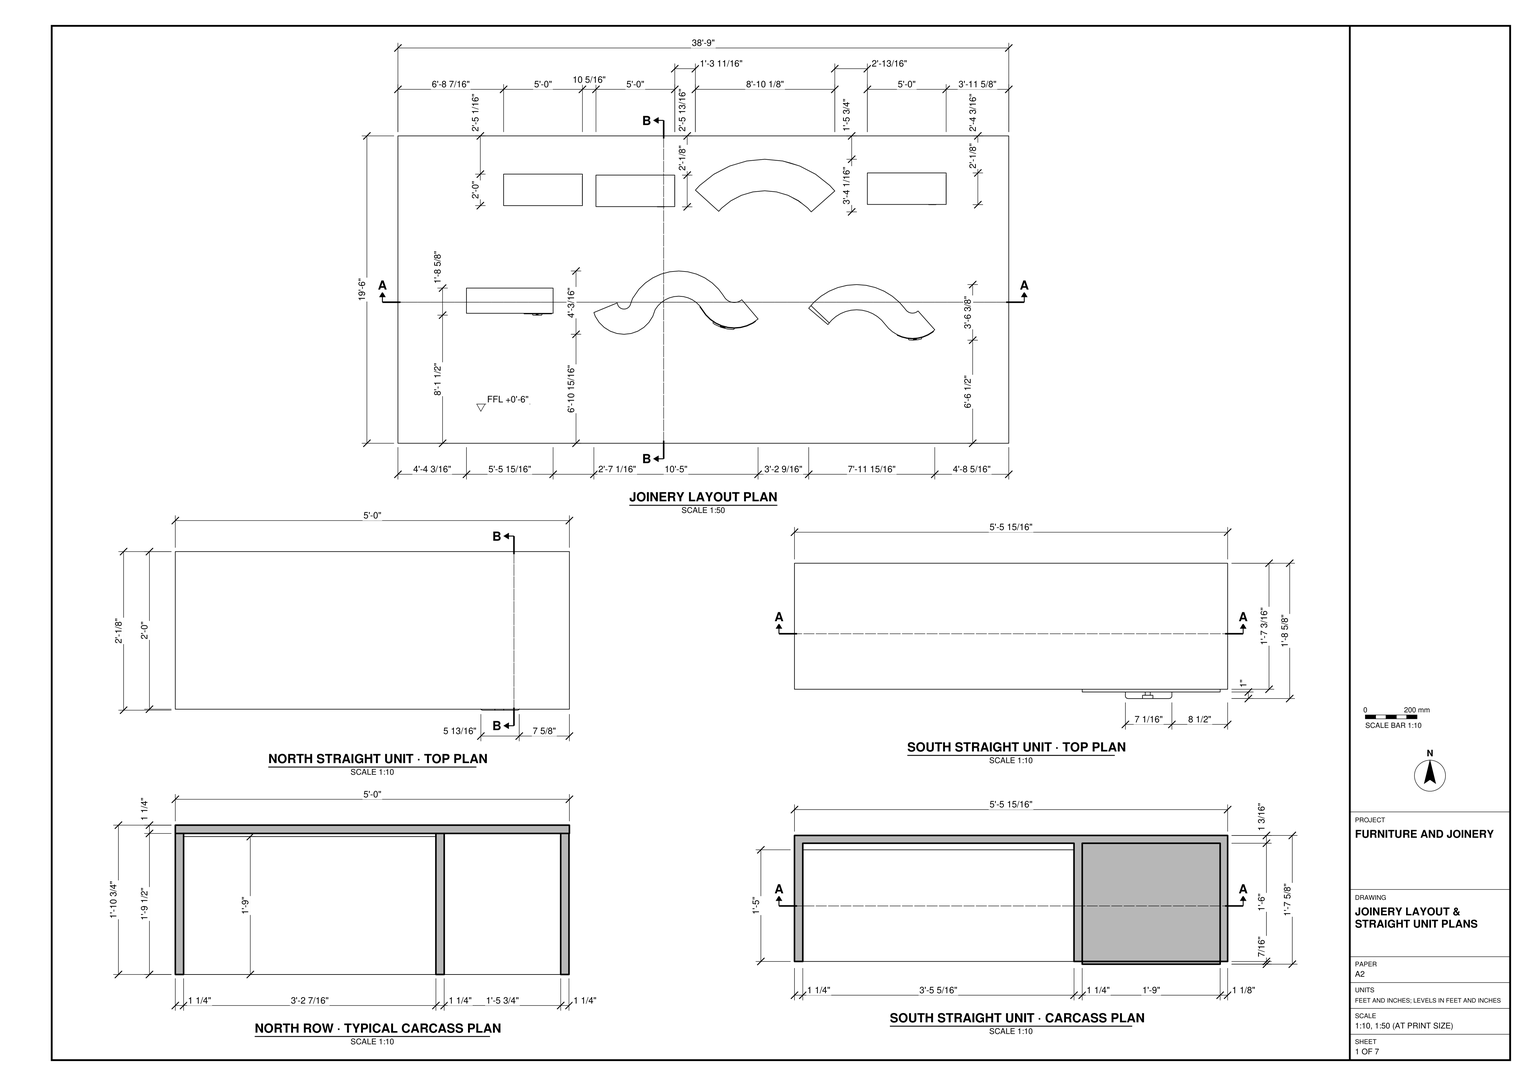
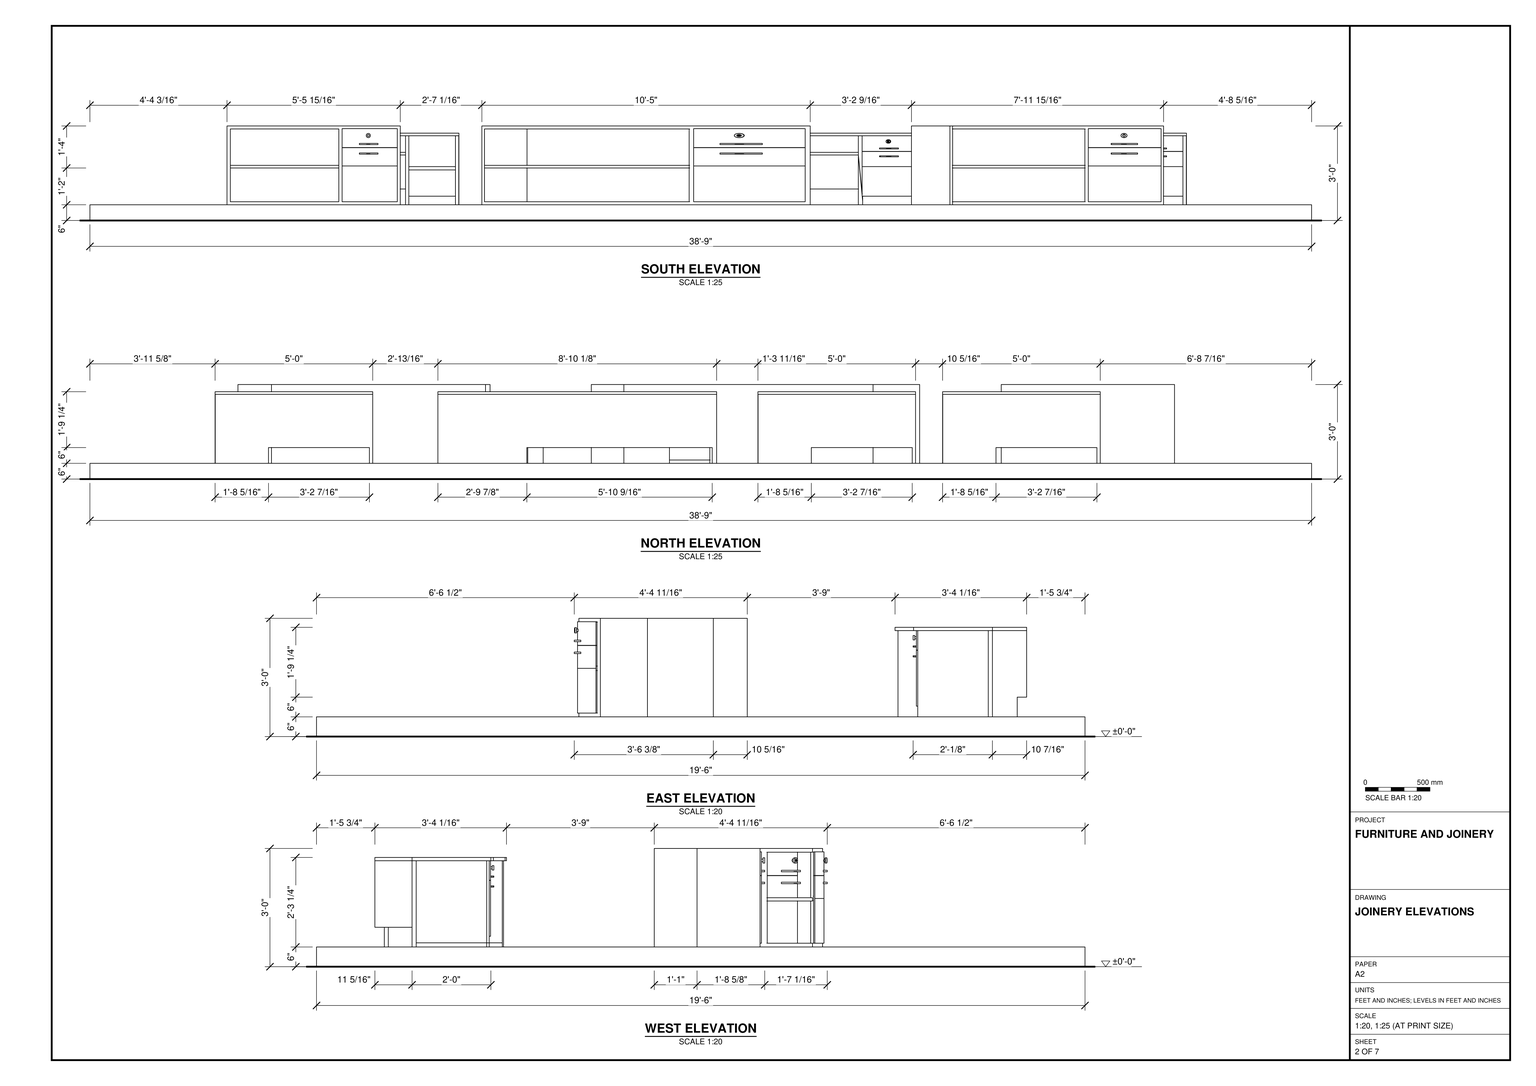
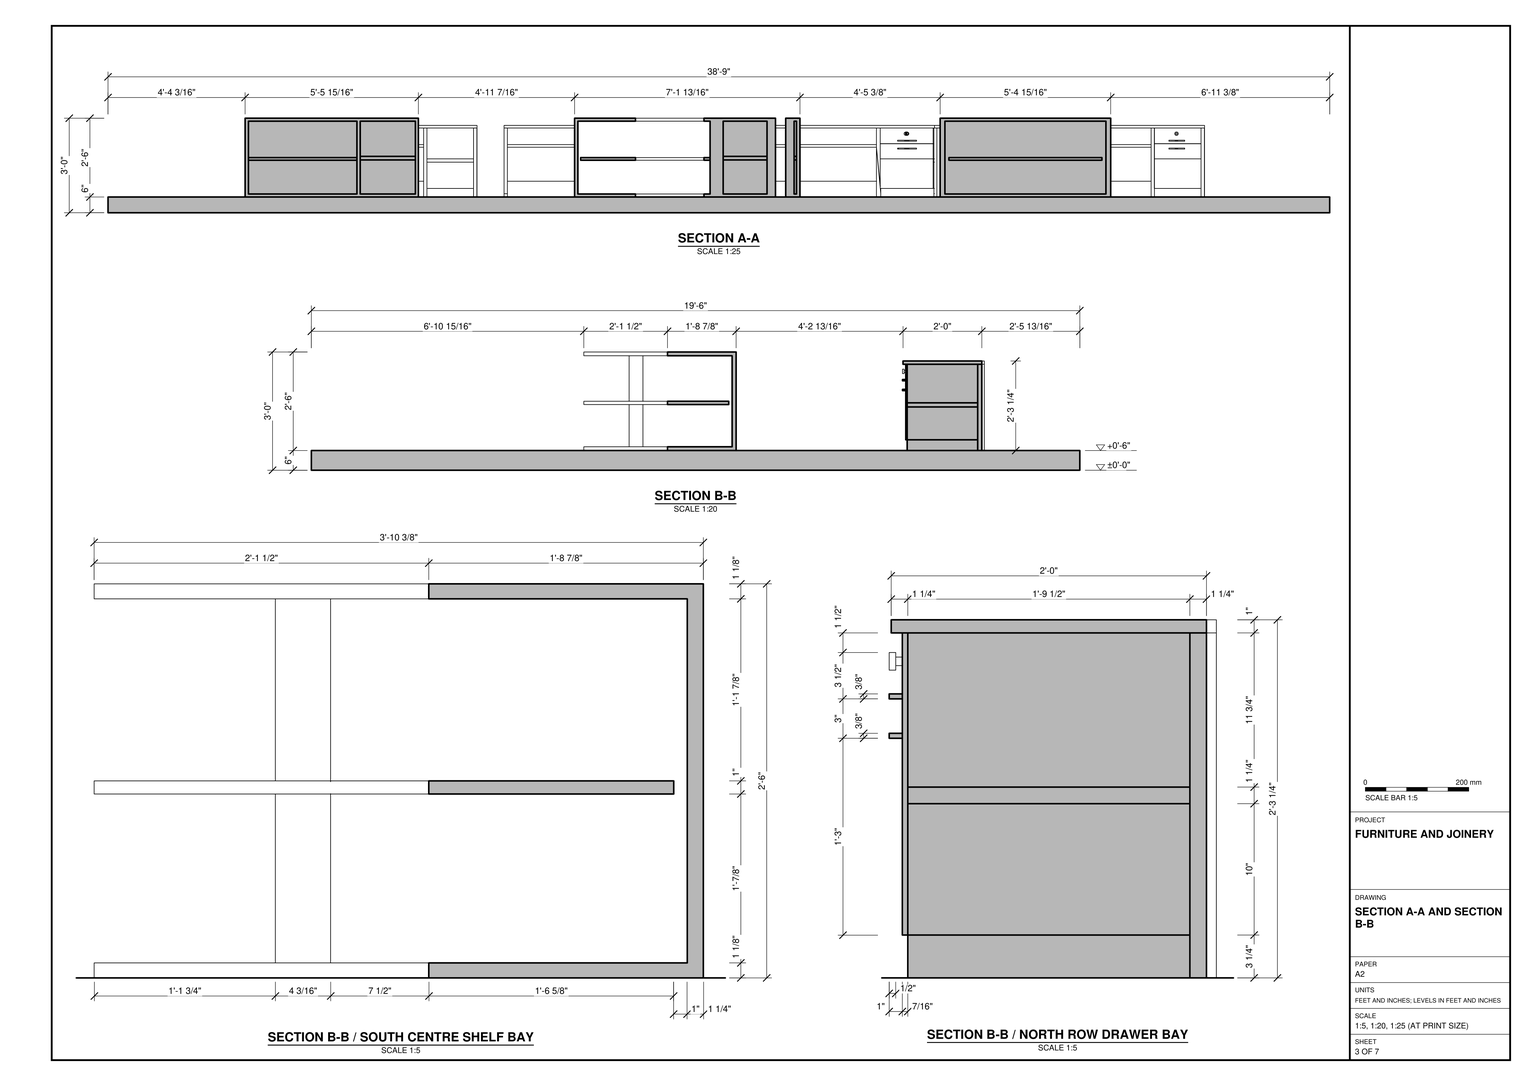
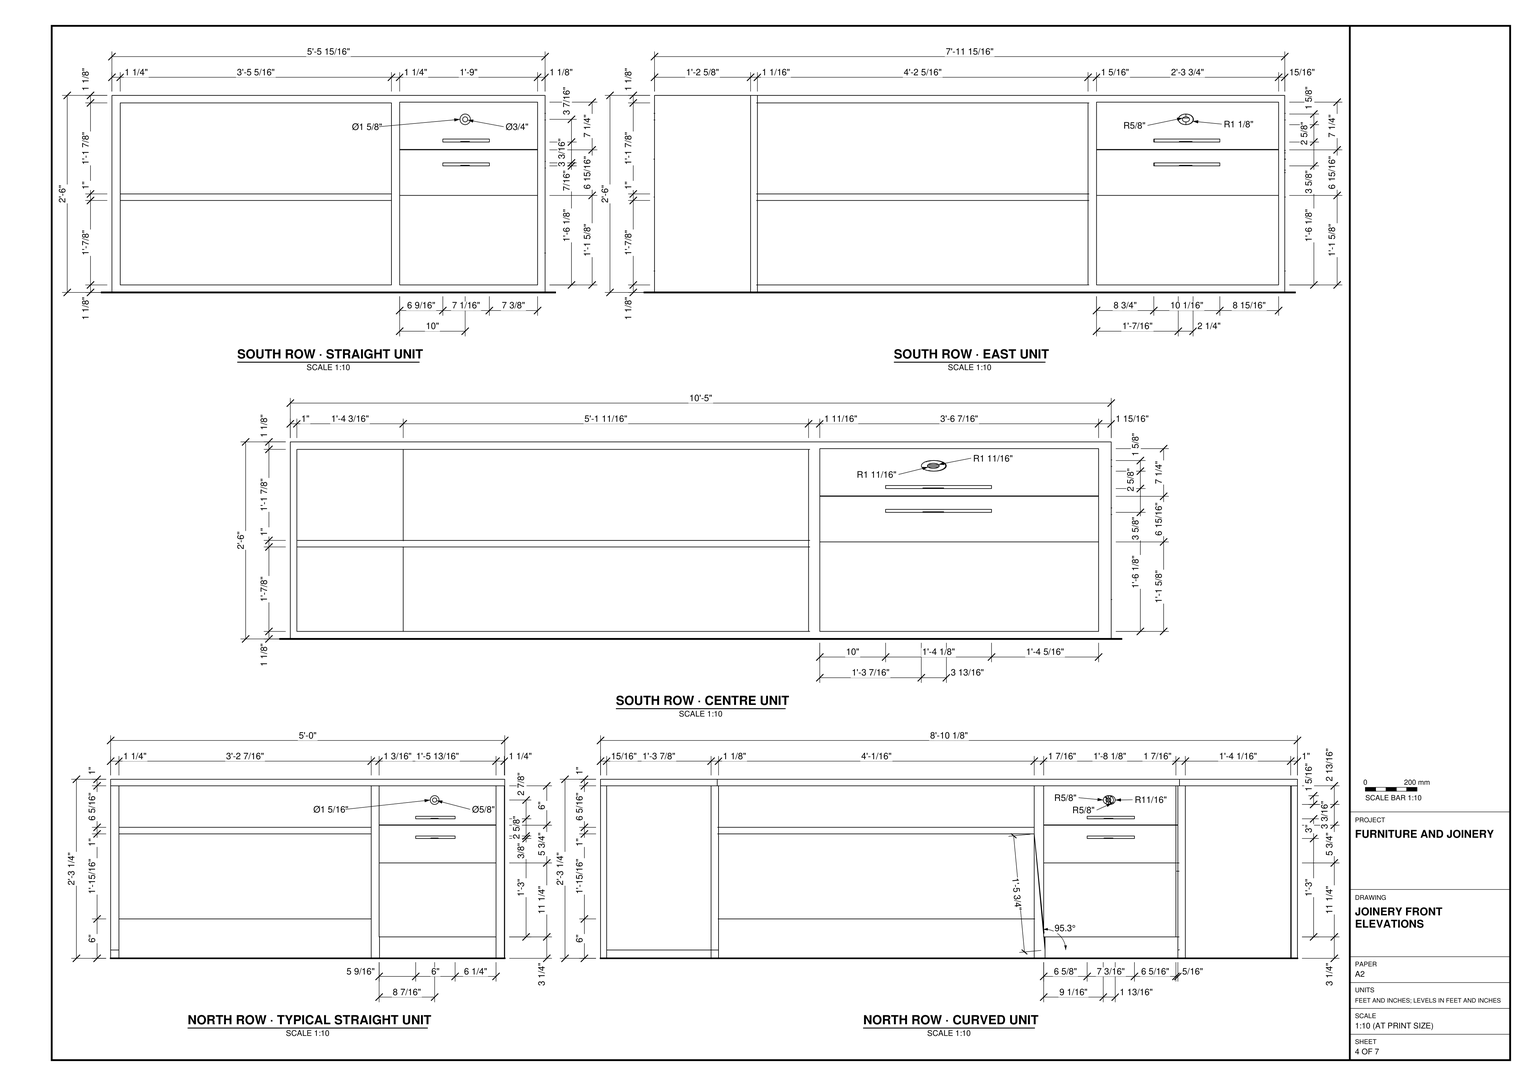
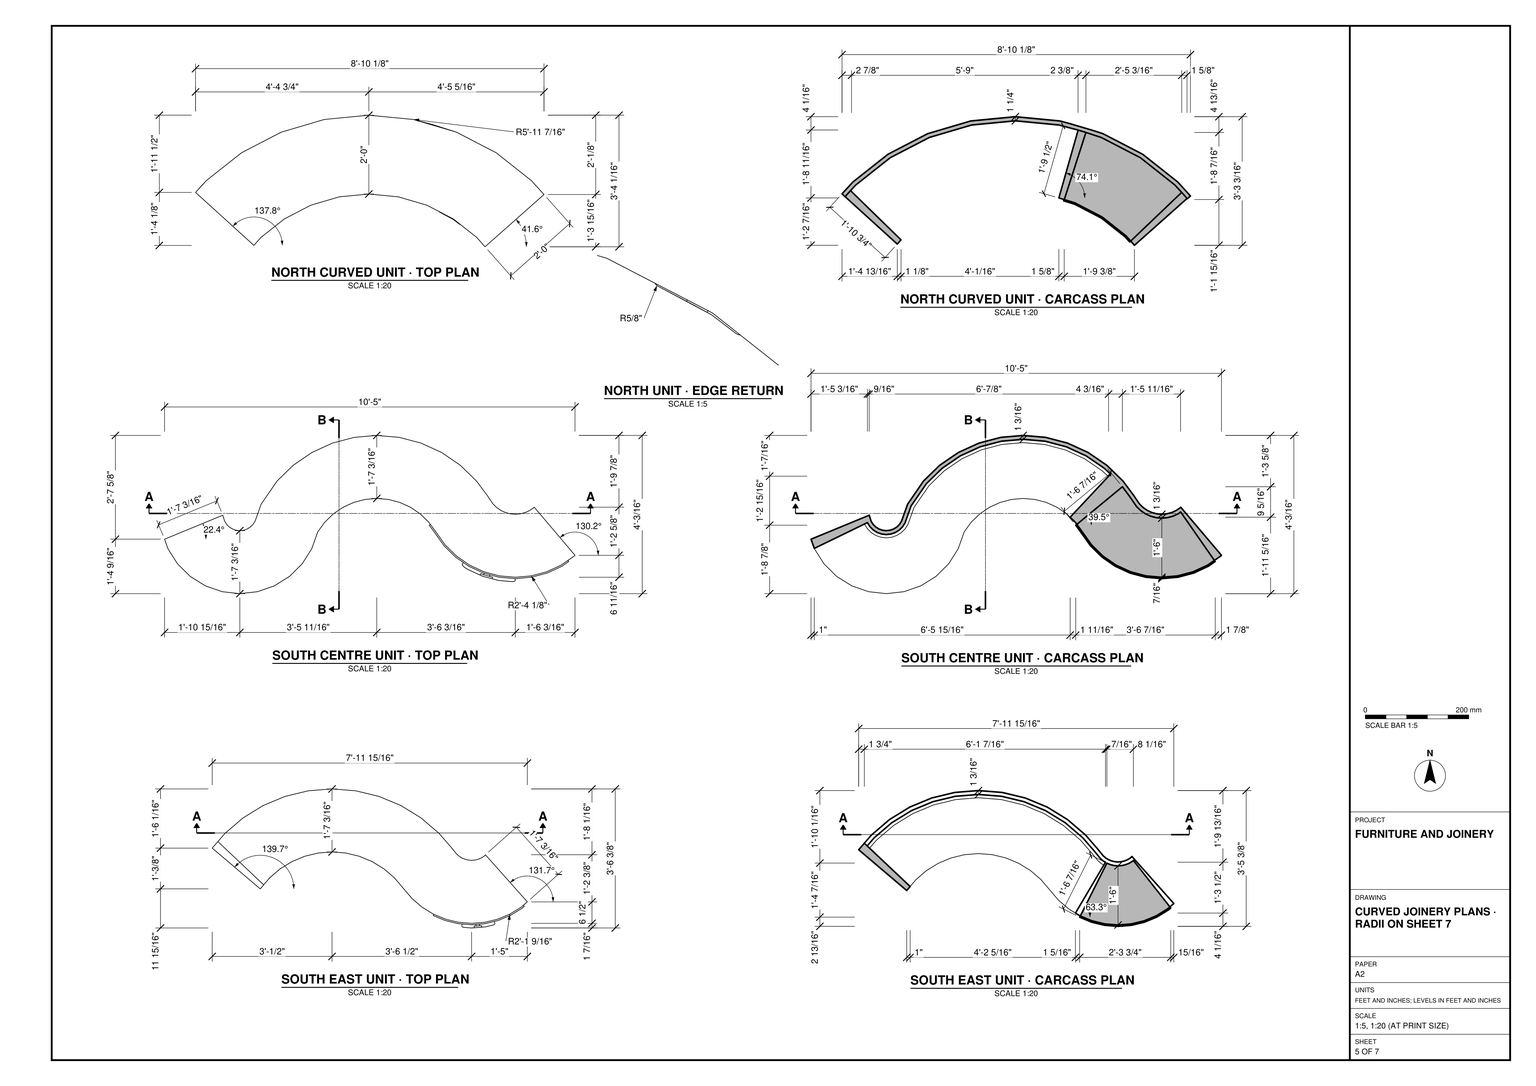
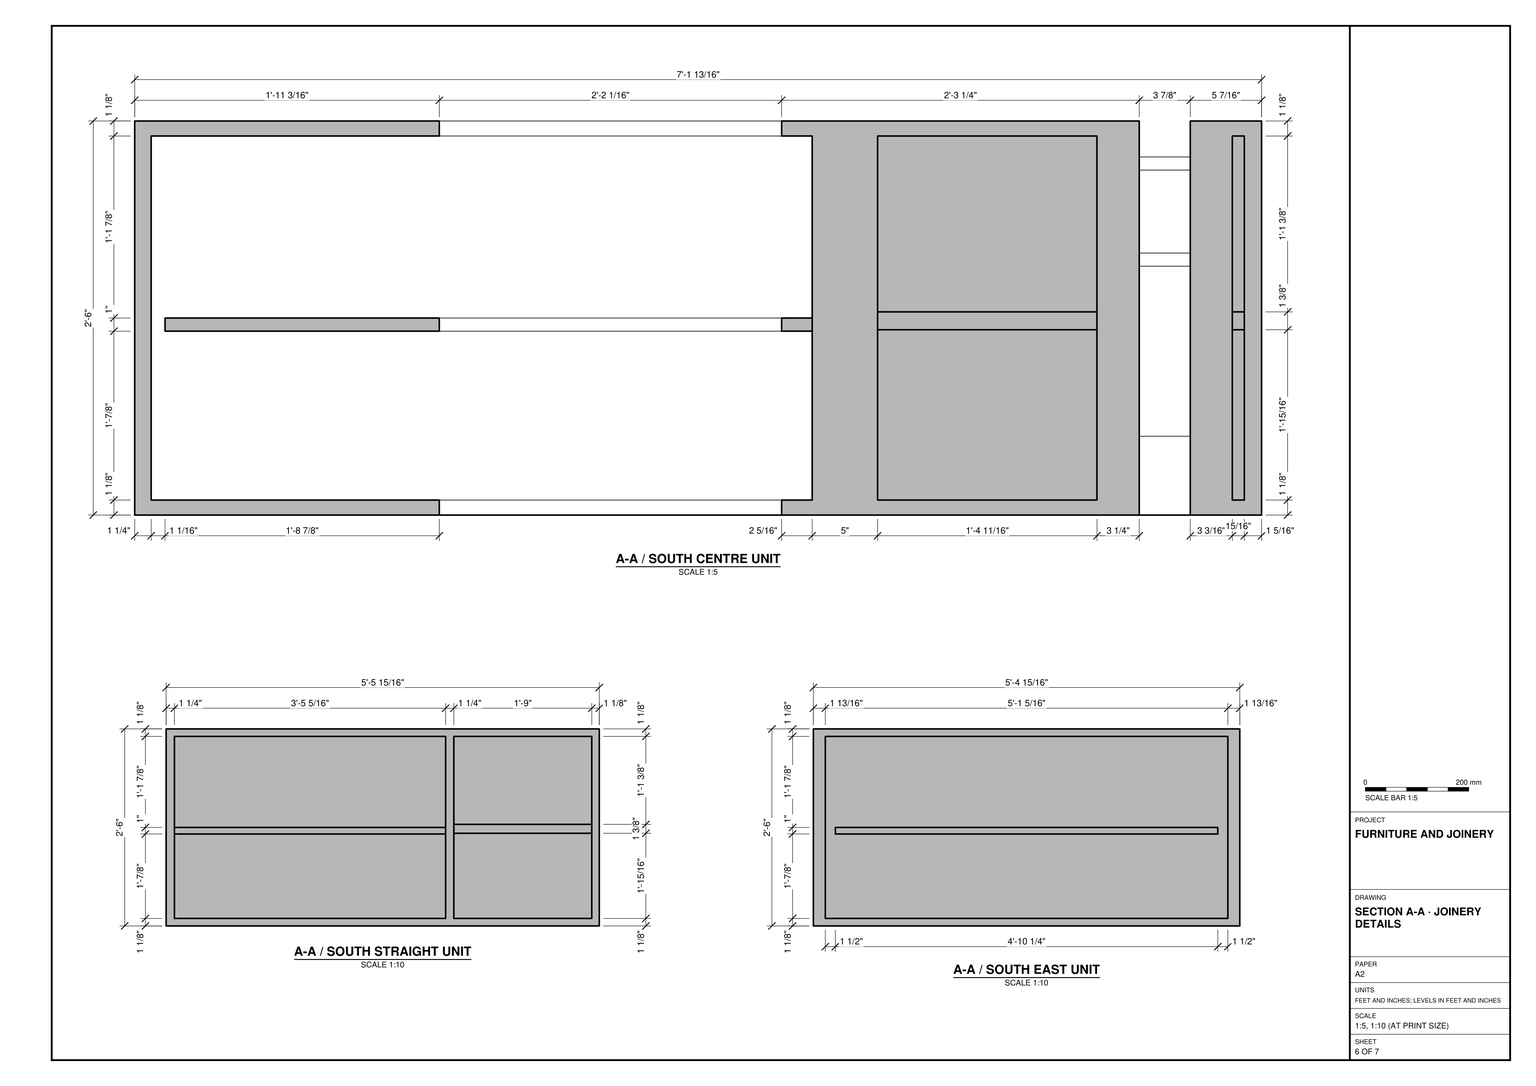
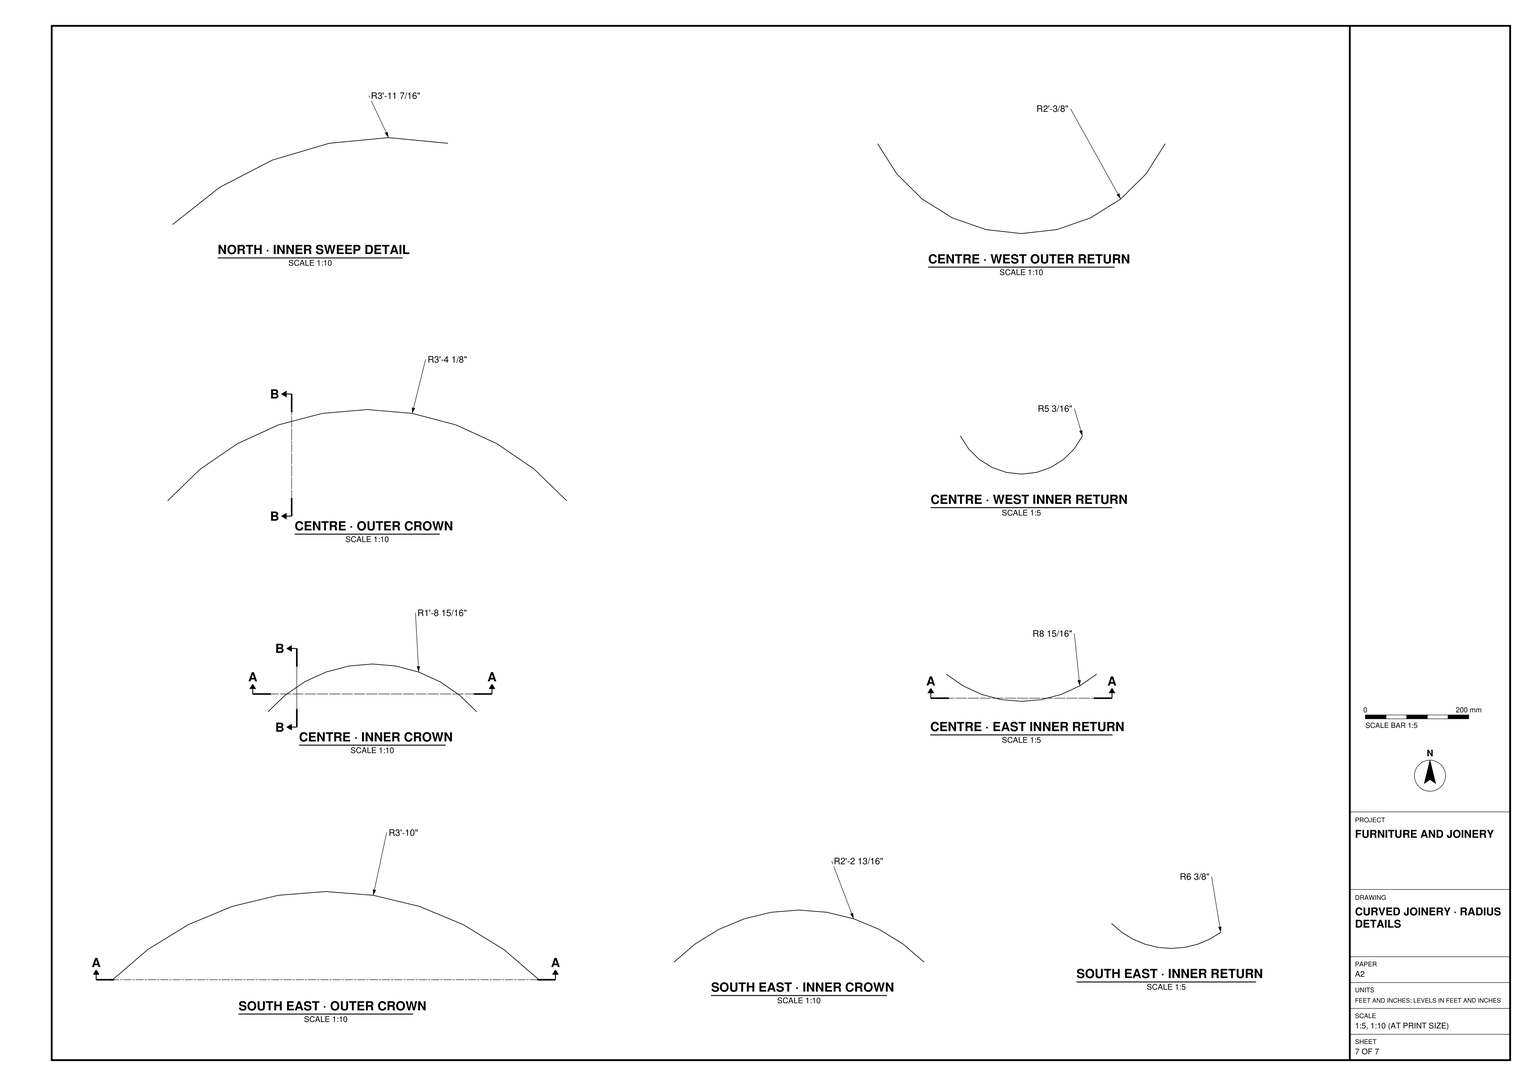
Build the joinery layout in SketchUp using task_files/diagram_01.pdf. Work in feet and inches. The overall model measures 38'-9" east to west, 19'-6" north to south and 3'-0" high. Use the underside of the rectangular slab as the datum at ±0'-0". The units stand on the slab at +0'-6".

Use the layout plan to position each unit, matching the gaps between units and the offsets from the slab edges. From west to east, the north row has two straight units, an arc-shaped unit and another straight unit. The south row starts with a straight unit, followed by a long wave-shaped unit and a shorter wave-shaped unit. Trace the inner and outer curves of each top in plan and use the sections to establish the height of each row above the slab.

Build the carcasses with distinct tops, sides, backs, dividers and shelves at the thicknesses shown. Keep the shelf bays open and reproduce the adjoining storage fronts and their hardware as drawn in elevation. Keep the slab and each joinery piece in separate groups or components, and use components for repeated parts. Decor and loose items, if shown, may be any suitable library components. Save one SketchUp model as output_files/straight_and_curved_storage_units_on_their_slab.skp.

# SketchUp Ruby script. Lengths in inches.
U = 1.inch
M = Sketchup.active_model
def pt(a) = Geom::Point3d.new(a.map { |v| v * U })
def face(e, loops, mat)
  f = e.add_face(loops[0].map { |a| pt(a) })
  loops[1..].each { |l| e.add_face(l.map { |a| pt(a) }).erase! }
  f.material = f.back_material = mat if mat
  f
end
# faces: each face lists its corners as indices into pts; further lists are holes
def faces(e, pts, list, mat = nil) = list.each { |f| face(e, (f[0].is_a?(Array) ? f : [f]).map { |l| l.map { |i| pts[i] } }, mat) }
# xy, xz, yz: faces in a plane at the given z, y or x. An outline is a flat list of corners, or four numbers for a rectangle; further outlines are holes
def ring(l) = l.size == 4 ? [[l[0], l[1]], [l[2], l[1]], [l[2], l[3]], [l[0], l[3]]] : l.each_slice(2).to_a
def flat(e, list, mat, &to3) = list.each { |f| face(e, (f[0].is_a?(Array) ? f : [f]).map { |l| ring(l).map { |u, v| to3.(u, v) } }, mat) }
def xy(e, z, list, mat = nil) = flat(e, list, mat) { |x, y| [x, y, z] }
def xz(e, y, list, mat = nil) = flat(e, list, mat) { |x, z| [x, y, z] }
def yz(e, x, list, mat = nil) = flat(e, list, mat) { |y, z| [x, y, z] }
def lines(e, pts, list) = list.each { |a, b| e.add_line(pt(pts[a]), pt(pts[b])) }
# prism: a flat outline (further loops are holes) pulled along v
def prism(e, loops, v, mat = nil)
  f = face(e, loops, mat); d = Geom::Vector3d.new(v.map { |x| x * U })
  f.pushpull(f.normal.samedirection?(d) ? d.length : -d.length)
end
def box(e, o, s, mat = nil) = prism(e, [[o, [o[0] + s[0], o[1], o[2]], [o[0] + s[0], o[1] + s[1], o[2]], [o[0], o[1] + s[1], o[2]]]], [0, 0, s[2]], mat)
def at(x, y, z, deg = 0) = Geom::Transformation.translation(pt([x, y, z])) * Geom::Transformation.rotation(ORIGIN, Z_AXIS, deg.degrees)
def axes(o, x, y, z) = Geom::Transformation.new([*x, 0, *y, 0, *z, 0, *pt(o).to_a, 1])
def part(name) = M.definitions.add(name)
# library, detail: a bought-in or finely detailed component or shape, given as its bounding box
def library(name, o, s) = part(name).tap { |d| box(d.entities, o, s) }
def detail(e, o, s) = box(e.add_group.entities, o, s)
def put(e, d, t, mat = nil) = e.add_instance(d, t).tap { |i| i.material = mat if mat }
def group(e, t, mat = nil) = e.add_group.tap { |g| g.transformation = t; g.material = mat if mat }.entities
root = M.entities
M.materials.add("[Color A01]").color = [204, 172, 120]
M.materials.add("[Color A01]1").color = [176, 88, 14]
M.materials.add("[Color E05]").color = [124, 72, 50]
M.materials.add("[Encaustic Tile Circular 02]").color = [187, 174, 162]
M.materials.add("[Wood Floor Light]").color = [204, 176, 127]
M.materials.add("[Wood Floor Light]1").color = [204, 176, 127]
c1 = part("Group\#10")
box(c1.entities,[0,0,0],[60,24,1],"[Color E05]")
c2 = part("Group\#8")
box(c2.entities,[58.74,-20.21,7.26],[1.26,21.47,17.74])
c3 = part("Group\#16")
box(c3.entities,[-5.41,3,0],[38.41,21,1],"[Color A01]")
c4 = part("Group\#5")
box(c4.entities,[56.74,-18.95,7.33],[3.26,21.48,17.73],"[Color E05]")
c5 = part("Group\#6")
box(c5.entities,[0,0,-3.26],[1.26,21.47,26.26],"[Color E05]")
c6 = part("Group\#2")
box(c6.entities,[0,0,-1.26],[1.26,21.47,1.26],"[Color E05]")
g1 = group(c6.entities,at(0,0,0))
xy(g1,25,[[0,0,1.26,21.47]],"[Color E05]")
xz(g1,0,[[0,0,1.26,25]],"[Color E05]")
xz(g1,21.47,[[0,0,1.26,25]],"[Color E05]")
yz(g1,0,[[0,0,21.47,25]],"[Color E05]")
yz(g1,1.26,[[0,0,21.47,25]],"[Color E05]")
c7 = part("Group\#1")
prism(c7.entities,[[[60,1.26,0],[39.67,1.26,0],[39.67,1.26,6],[39.26,1.26,6],[1.26,1.26,6],[1.26,1.26,0],[0,1.26,0],[0,1.26,26.26],[60,1.26,26.26]]],[0,-1.26,0],"[Color E05]")
c8 = part("Group\#4")
box(c8.entities,[0,0,-3.26],[1.26,21.47,26.26],"[Color E05]")
c9 = part("Group\#12")
xy(c9.entities,0,[[0.33,0,0.28,0.01,0.23,0.03,0.19,0.05,0.11,0.11,0.05,0.19,0.03,0.23,0.01,0.28,0,0.33,0,1,2.3,1,2.29,0],[2.29,0,2.3,1,2.3,0],[2.3,0,3.43,0.13],[3.43,0,3.43,1,6,1,6,0.35,5.99,0.3,5.95,0.2,5.92,0.16,5.84,0.08,5.8,0.05,5.7,0.01,5.65,0]],"[Color E05]")
xy(c9.entities,0.2,[[2.3,0.13,3.43,1]],"[Color E05]")
xy(c9.entities,1,[[0.33,0,5.65,0,5.7,0.01,5.8,0.05,5.84,0.08,5.92,0.16,5.95,0.2,5.99,0.3,6,0.35,6,1,0,1,0,0.33,0.01,0.28,0.03,0.23,0.05,0.19,0.11,0.11,0.19,0.05,0.23,0.03,0.28,0.01]],"[Color E05]")
xz(c9.entities,0,[[0.33,0,0.38,1],[0.38,0,5.6,1],[5.6,0,5.65,1]],"[Color E05]")
xz(c9.entities,0.13,[[2.3,0,3.43,0.2]],"[Color E05]")
xz(c9.entities,1,[[0,0,2.3,1],[3.43,0,6,1],[2.3,0.2,3.43,1]],"[Color E05]")
yz(c9.entities,0,[[0.33,0,0.38,1],[0.38,0,1,1]],"[Color E05]")
yz(c9.entities,2.3,[[0.13,0,1,0.2]],"[Color E05]")
yz(c9.entities,3.43,[[0.13,0,1,0.2]],"[Color E05]")
yz(c9.entities,6,[[0.35,0,0.4,1],[0.4,0,1,1]],"[Color E05]")
p = [[0.19,0.05,0],[0.23,0.03,0],[0.23,0.03,1],[0.19,0.05,1],[0.28,0.01,0],[0.28,0.01,1],
  [0.33,0,0],[0.33,0,1],[5.65,0,0],[5.7,0.01,0],[5.7,0.01,1],[5.65,0,1],
  [5.75,0.03,0],[5.75,0.03,1],[5.8,0.05,0],[5.8,0.05,1],[0.11,0.11,0],[0.15,0.08,0],
  [0.15,0.08,1],[0.11,0.11,1],[0.08,0.15,0],[0.08,0.15,1],[0.05,0.19,0],[0.05,0.19,1],
  [5.84,0.08,0],[5.88,0.12,0],[5.88,0.12,1],[5.84,0.08,1],[5.92,0.16,0],[5.92,0.16,1],
  [0.01,0.28,0],[0.03,0.23,0],[0.03,0.23,1],[0.01,0.28,1],[5.95,0.2,0],[5.95,0.2,1],
  [5.97,0.25,0],[5.97,0.25,1],[5.99,0.3,0],[5.99,0.3,1],[0,0.33,0],[0,0.33,1],
  [6,0.35,0],[6,0.35,1],[3.43,0.13,0.2],[3.43,0,0.2],[2.3,0,0.2],[2.3,0.13,0.2]]
faces(c9.entities,p,[[0,1,2,3],[1,4,5,2],[4,6,7,5],[8,9,10,11],[9,12,13,10],[12,14,15,13],[16,17,18,19],[17,0,3,18],
  [20,16,19,21],[22,20,21,23],[24,25,26,27],[14,24,27,15],[25,28,29,26],[30,31,32,33],[31,22,23,32],[28,34,35,29],
  [34,36,37,35],[36,38,39,37],[40,30,33,41],[38,42,43,39]],"[Color E05]")
lines(c9.entities,p,[[44,45],[46,47]])
c10 = part("Group\#11")
xy(c10.entities,0,[[0.33,0,0.28,0.01,0.23,0.03,0.19,0.05,0.11,0.11,0.05,0.19,0.03,0.23,0.01,0.28,0,0.33,0,1,2.3,1,2.29,0],[2.29,0,2.3,1,2.3,0],[2.3,0,3.43,0.13],[3.43,0,3.43,1,6,1,6,0.35,5.99,0.3,5.95,0.2,5.92,0.16,5.84,0.08,5.8,0.05,5.7,0.01,5.65,0]],"[Color A01]")
xy(c10.entities,0.2,[[2.3,0.13,3.43,1]],"[Color A01]")
xy(c10.entities,1,[[0.33,0,5.65,0,5.7,0.01,5.8,0.05,5.84,0.08,5.92,0.16,5.95,0.2,5.99,0.3,6,0.35,6,1,0,1,0,0.33,0.01,0.28,0.03,0.23,0.05,0.19,0.11,0.11,0.19,0.05,0.23,0.03,0.28,0.01]],"[Color A01]")
xz(c10.entities,0,[[0.33,0,0.38,1],[0.38,0,5.6,1],[5.6,0,5.65,1]],"[Color A01]")
xz(c10.entities,0.13,[[2.3,0,3.43,0.2]],"[Color A01]")
xz(c10.entities,1,[[0,0,2.3,1],[3.43,0,6,1],[2.3,0.2,3.43,1]],"[Color A01]")
yz(c10.entities,0,[[0.33,0,0.38,1],[0.38,0,1,1]],"[Color A01]")
yz(c10.entities,2.3,[[0.13,0,1,0.2]],"[Color A01]")
yz(c10.entities,3.43,[[0.13,0,1,0.2]],"[Color A01]")
yz(c10.entities,6,[[0.35,0,0.4,1],[0.4,0,1,1]],"[Color A01]")
p = [[0.23,0.03,0],[0.28,0.01,0],[0.28,0.01,1],[0.23,0.03,1],[0.19,0.05,0],[0.19,0.05,1],
  [0.33,0,0],[0.33,0,1],[5.65,0,0],[5.7,0.01,0],[5.7,0.01,1],[5.65,0,1],
  [5.75,0.03,0],[5.75,0.03,1],[5.8,0.05,0],[5.8,0.05,1],[0.08,0.15,0],[0.11,0.11,0],
  [0.11,0.11,1],[0.08,0.15,1],[0.05,0.19,0],[0.05,0.19,1],[0.15,0.08,0],[0.15,0.08,1],
  [5.84,0.08,0],[5.84,0.08,1],[5.88,0.12,0],[5.88,0.12,1],[5.92,0.16,0],[5.92,0.16,1],
  [0.01,0.28,0],[0.03,0.23,0],[0.03,0.23,1],[0.01,0.28,1],[5.95,0.2,0],[5.97,0.25,0],
  [5.97,0.25,1],[5.95,0.2,1],[5.99,0.3,0],[5.99,0.3,1],[0,0.33,0],[0,0.33,1],
  [6,0.35,0],[6,0.35,1],[3.43,0.13,0.2],[3.43,0,0.2],[2.3,0,0.2],[2.3,0.13,0.2]]
faces(c10.entities,p,[[0,1,2,3],[4,0,3,5],[1,6,7,2],[8,9,10,11],[9,12,13,10],[12,14,15,13],[16,17,18,19],[20,16,19,21],
  [17,22,23,18],[22,4,5,23],[14,24,25,15],[24,26,27,25],[26,28,29,27],[30,31,32,33],[31,20,21,32],[34,35,36,37],
  [28,34,37,29],[35,38,39,36],[40,30,33,41],[38,42,43,39]],"[Color A01]")
lines(c10.entities,p,[[44,45],[46,47]])
c11 = part("Straight storage unit")
p = [[1.26,22.89,1.26],[1.26,22.89,8.26],[40.9375,1.42,1.26],[40.9375,3.15,1.63],[58.74,3.15,1.63],[58.74,1.42,1.26]]
lines(c11.entities,p,[[0,1],[2,3],[4,5]])
put(c11.entities,c1,at(0,0.15,26.26),"[Color A01]")
put(c11.entities,c2,axes([33.67,21.63,73.26],[0,0,-1],[0,1,0],[1,0,0]),"[Color A01]")
put(c11.entities,c3,at(6.67,-1.58,18.95),"[Color A01]")
put(c11.entities,c4,axes([33.61,20.37,60],[0,0,-1],[0,1,0],[1,0,0]),"[Color E05]")
put(c11.entities,c5,at(39.67,1.42,3.26),"[Color E05]")
put(c11.entities,c6,at(0,1.42,1.26),"[Color E05]")
put(c11.entities,c7,at(0,22.89,0),"[Color E05]")
put(c11.entities,c8,at(58.67,1.42,3.26),"[Color E05]")
g2 = group(c11.entities,at(40.875,0,3.26))
xy(g2,0,[[0,1,17.8,1.42]],"[Color E05]")
xy(g2,23,[[0,1,17.8,1.42]],"[Color E05]")
xz(g2,0,[[[8.45,20.17,8.625,20.1875,8.79,20.26,8.93,20.36,9.03,20.5,9.1,20.66,9.125,20.84,9.1,21.01,9.03,21.17,8.93,21.3125,8.79,21.42,8.625,21.49,8.45,21.51,8.28,21.49,8.12,21.42,7.98,21.3125,7.87,21.17,7.8,21.01,7.78,20.84,7.8,20.66,7.87,20.5,7.98,20.36,8.12,20.26,8.28,20.1875],[8.45,20.51,8.37,20.52,8.29,20.56,8.22,20.61,8.17,20.68,8.14,20.75,8.13,20.84,8.14,20.92,8.17,21,8.22,21.07,8.29,21.12,8.37,21.15,8.45,21.16,8.54,21.15,8.62,21.12,8.68,21.07,8.73,21,8.77,20.92,8.78,20.84,8.77,20.75,8.73,20.68,8.68,20.61,8.62,20.56,8.54,20.52]],[8.45,20.51,8.54,20.52,8.62,20.56,8.68,20.61,8.73,20.68,8.77,20.75,8.78,20.84,8.77,20.92,8.73,21,8.68,21.07,8.62,21.12,8.54,21.15,8.45,21.16,8.37,21.15,8.29,21.12,8.22,21.07,8.17,21,8.14,20.92,8.13,20.84,8.14,20.75,8.17,20.68,8.22,20.61,8.29,20.56,8.37,20.52]],"[Color E05]")
xz(g2,0.5,[[[8.45,20.17,8.625,20.1875,8.79,20.26,8.93,20.36,9.03,20.5,9.1,20.66,9.125,20.84,9.1,21.01,9.03,21.17,8.93,21.3125,8.79,21.42,8.625,21.49,8.45,21.51,8.28,21.49,8.12,21.42,7.98,21.3125,7.87,21.17,7.8,21.01,7.78,20.84,7.8,20.66,7.87,20.5,7.98,20.36,8.12,20.26,8.28,20.1875],[8.45,20.51,8.37,20.52,8.29,20.56,8.22,20.61,8.17,20.68,8.14,20.75,8.13,20.84,8.14,20.92,8.17,21,8.22,21.07,8.29,21.12,8.37,21.15,8.45,21.16,8.54,21.15,8.62,21.12,8.68,21.07,8.73,21,8.77,20.92,8.78,20.84,8.77,20.75,8.73,20.68,8.68,20.61,8.62,20.56,8.54,20.52]]],"[Color E05]")
xz(g2,1,[[0,0,17.8,11.26],[0,11.26,17.8,17],[[0,17.05,17.8,23],[8.45,20.51,8.37,20.52,8.29,20.56,8.22,20.61,8.17,20.68,8.14,20.75,8.13,20.84,8.14,20.92,8.17,21,8.22,21.07,8.29,21.12,8.37,21.15,8.45,21.16,8.54,21.15,8.62,21.12,8.68,21.07,8.73,21,8.77,20.92,8.78,20.84,8.77,20.75,8.73,20.68,8.68,20.61,8.62,20.56,8.54,20.52]]],"[Color A01]")
xz(g2,1,[[0,17,17.8,17.05],[8.45,20.51,8.54,20.52,8.62,20.56,8.68,20.61,8.73,20.68,8.77,20.75,8.78,20.84,8.77,20.92,8.73,21,8.68,21.07,8.62,21.12,8.54,21.15,8.45,21.16,8.37,21.15,8.29,21.12,8.22,21.07,8.17,21,8.14,20.92,8.13,20.84,8.14,20.75,8.17,20.68,8.22,20.61,8.29,20.56,8.37,20.52]],"[Color E05]")
xz(g2,1.42,[[0,0,17.8,23]],"[Color E05]")
yz(g2,0,[[1,0,1.42,17],[1,17,1.42,17.05],[1,17.05,1.42,23]],"[Color E05]")
yz(g2,17.8,[[1,0,1.42,17],[1,17,1.42,17.05],[1,17.05,1.42,23]],"[Color E05]")
p = [[8.28,0,20.1875],[8.12,0,20.26],[8.12,0.5,20.26],[8.28,0.5,20.1875],[8.45,0,20.17],[8.45,0.5,20.17],
  [8.625,0,20.1875],[8.625,0.5,20.1875],[8.79,0,20.26],[8.79,0.5,20.26],[7.98,0,20.36],[7.98,0.5,20.36],
  [8.93,0,20.36],[8.93,0.5,20.36],[7.87,0,20.5],[7.87,0.5,20.5],[9.03,0,20.5],[9.03,0.5,20.5],
  [7.8,0,20.66],[7.8,0.5,20.66],[8.37,0,20.52],[8.29,0,20.56],[8.29,0.5,20.56],[8.37,0.5,20.52],
  [8.45,0,20.51],[8.45,0.5,20.51],[8.62,0,20.56],[8.54,0,20.52],[8.54,0.5,20.52],[8.62,0.5,20.56],
  [9.1,0,20.66],[9.1,0.5,20.66],[8.29,1,20.56],[8.37,1,20.52],[8.45,1,20.51],[8.54,1,20.52],
  [8.62,1,20.56],[8.22,0,20.61],[8.17,0,20.68],[8.17,0.5,20.68],[8.22,0.5,20.61],[8.68,0,20.61],
  [8.68,0.5,20.61],[8.73,0,20.68],[8.73,0.5,20.68],[8.17,1,20.68],[8.22,1,20.61],[8.68,1,20.61],
  [8.73,1,20.68],[7.78,0,20.84],[7.78,0.5,20.84],[8.14,0,20.75],[8.14,0.5,20.75],[8.77,0,20.75],
  [8.77,0.5,20.75],[9.125,0,20.84],[9.125,0.5,20.84],[8.14,1,20.75],[8.77,1,20.75],[7.8,0,21.01],
  [7.8,0.5,21.01],[8.13,0,20.84],[8.14,0,20.92],[8.14,0.5,20.92],[8.13,0.5,20.84],[8.78,0,20.84],
  [8.78,0.5,20.84],[8.77,0,20.92],[8.77,0.5,20.92],[9.1,0,21.01],[9.1,0.5,21.01],[8.13,1,20.84],
  [8.14,1,20.92],[8.78,1,20.84],[8.77,1,20.92],[8.17,0,21],[8.17,0.5,21],[8.73,0,21],
  [8.73,0.5,21],[8.17,1,21],[8.73,1,21],[7.87,0,21.17],[7.87,0.5,21.17],[8.22,0,21.07],
  [8.22,0.5,21.07],[8.68,0,21.07],[8.68,0.5,21.07],[9.03,0,21.17],[9.03,0.5,21.17],[8.22,1,21.07],
  [8.68,1,21.07],[8.29,0,21.12],[8.29,0.5,21.12],[8.37,0,21.15],[8.37,0.5,21.15],[8.54,0,21.15],
  [8.62,0,21.12],[8.62,0.5,21.12],[8.54,0.5,21.15],[8.29,1,21.12],[8.37,1,21.15],[8.62,1,21.12],
  [8.54,1,21.15],[7.98,0,21.3125],[7.98,0.5,21.3125],[8.45,0,21.16],[8.45,0.5,21.16],[8.93,0,21.3125],
  [8.93,0.5,21.3125],[8.45,1,21.16],[8.12,0,21.42],[8.12,0.5,21.42],[8.79,0,21.42],[8.79,0.5,21.42],
  [8.28,0,21.49],[8.28,0.5,21.49],[8.625,0,21.49],[8.625,0.5,21.49],[8.45,0,21.51],[8.45,0.5,21.51]]
faces(g2,p,[[0,1,2,3],[4,0,3,5],[6,4,5,7],[8,6,7,9],[1,10,11,2],[12,8,9,13],[10,14,15,11],[16,12,13,17],
  [14,18,19,15],[20,21,22,23],[24,20,23,25],[26,27,28,29],[27,24,25,28],[30,16,17,31],[32,33,23,22],[33,34,25,23],
  [34,35,28,25],[35,36,29,28],[37,38,39,40],[21,37,40,22],[41,26,29,42],[43,41,42,44],[45,46,40,39],[46,32,22,40],
  [36,47,42,29],[47,48,44,42],[18,49,50,19],[38,51,52,39],[53,43,44,54],[55,30,31,56],[57,45,39,52],[48,58,54,44],
  [49,59,60,50],[61,62,63,64],[51,61,64,52],[65,53,54,66],[67,65,66,68],[69,55,56,70],[71,57,52,64],[72,71,64,63],
  [73,74,68,66],[58,73,66,54],[62,75,76,63],[77,67,68,78],[79,72,63,76],[74,80,78,68],[59,81,82,60],[75,83,84,76],
  [85,77,78,86],[87,69,70,88],[89,79,76,84],[80,90,86,78],[83,91,92,84],[91,93,94,92],[95,96,97,98],[96,85,86,97],
  [99,89,84,92],[100,99,92,94],[101,102,98,97],[90,101,97,86],[81,103,104,82],[93,105,106,94],[105,95,98,106],[107,87,88,108],
  [109,100,94,106],[102,109,106,98],[103,110,111,104],[112,107,108,113],[110,114,115,111],[116,112,113,117],[114,118,119,115],[118,116,117,119]],"[Color E05]")
put(g2,c9,axes([5.57,0,17.98],[1,0,0],[0,1,0],[0,0,0.38]),"[Color A01]")
put(g2,c10,axes([5.57,0,14.98],[1,0,0],[0,1,0],[0,0,0.38]),"[Color A01]")
c12 = library("Shape Bender Component\#1",[0,0,0],[106.11,40.07,27.26])
c13 = library("Shape Bender Component\#2",[0,0,0],[95.96,42.35,30])
c14 = part("Curved storage unit")
xy(c14.entities,0,[[0,1.42,65.95,20.6]],"[Color A01]1")
xy(c14.entities,1.14,[[1.27,1.42,42.56,19.42],[43.81,1.42,64.81,19.42]],"[Color A01]1")
xy(c14.entities,14.11,[[43.81,1.42,64.81,19.42]],"[Color A01]1")
xy(c14.entities,15.47,[[43.81,1.42,64.81,19.42]],"[Color A01]1")
xy(c14.entities,28.86,[[1.27,1.42,42.56,19.42],[43.81,1.42,64.81,19.42]],"[Color A01]1")
xy(c14.entities,30,[[0,1.42,65.95,20.6]],"[Color A01]1")
xz(c14.entities,1.42,[[[0,0,65.95,30],[1.27,1.14,42.56,28.86],[43.81,1.14,64.81,28.86]],[43.81,14.11,64.81,15.47]],"[Color A01]1")
xz(c14.entities,19.42,[[43.81,14.11,64.81,15.47]])
xz(c14.entities,19.42,[[1.27,1.14,42.56,28.86],[43.81,1.14,64.81,14.11],[43.81,15.47,64.81,28.86]],"[Color A01]1")
xz(c14.entities,20.6,[[0,0,65.95,30]],"[Color A01]1")
yz(c14.entities,0,[[1.42,0,20.6,30]],"[Color A01]1")
yz(c14.entities,1.27,[[1.42,1.14,19.42,28.86]],"[Color A01]1")
yz(c14.entities,42.56,[[1.42,1.14,19.42,28.86]],"[Color A01]1")
yz(c14.entities,43.81,[[1.42,14.11,19.42,15.47]])
yz(c14.entities,43.81,[[1.42,1.14,19.42,14.11],[1.42,15.47,19.42,28.86]],"[Color A01]1")
yz(c14.entities,64.81,[[1.42,14.11,19.42,15.47]])
yz(c14.entities,64.81,[[1.42,1.14,19.42,14.11],[1.42,15.47,19.42,28.86]],"[Color A01]1")
yz(c14.entities,65.95,[[1.42,0,20.6,30]],"[Color A01]1")
g3 = group(c14.entities,at(43.81,0,1.14),"[Wood Floor Light]")
xy(g3,0,[[0,1,21,1.42]],"[Wood Floor Light]")
xy(g3,27.83,[[0,1,21,1.42]],"[Wood Floor Light]")
xz(g3,0,[[[9.97,24.4,10.18,24.43,10.37,24.51,10.53,24.64,10.66,24.81,10.74,25,10.76,25.21,10.74,25.42,10.66,25.62,10.53,25.79,10.37,25.92,10.18,26,9.97,26.03,9.77,26,9.58,25.92,9.41,25.79,9.29,25.62,9.21,25.42,9.18,25.21,9.21,25,9.29,24.81,9.41,24.64,9.58,24.51,9.77,24.43],[9.97,24.82,9.875,24.83,9.78,24.875,9.7,24.9375,9.64,25.02,9.6,25.11,9.59,25.21,9.6,25.32,9.64,25.41,9.7,25.49,9.78,25.55,9.875,25.59,9.97,25.61,10.07,25.59,10.16,25.55,10.24,25.49,10.3,25.41,10.34,25.32,10.36,25.21,10.34,25.11,10.3,25.02,10.24,24.9375,10.16,24.875,10.07,24.83]],[9.97,24.82,10.07,24.83,10.16,24.875,10.24,24.9375,10.3,25.02,10.34,25.11,10.36,25.21,10.34,25.32,10.3,25.41,10.24,25.49,10.16,25.55,10.07,25.59,9.97,25.61,9.875,25.59,9.78,25.55,9.7,25.49,9.64,25.41,9.6,25.32,9.59,25.21,9.6,25.11,9.64,25.02,9.7,24.9375,9.78,24.875,9.875,24.83]],"[Wood Floor Light]")
xz(g3,0.5,[[[9.97,24.4,10.18,24.43,10.37,24.51,10.53,24.64,10.66,24.81,10.74,25,10.76,25.21,10.74,25.42,10.66,25.62,10.53,25.79,10.37,25.92,10.18,26,9.97,26.03,9.77,26,9.58,25.92,9.41,25.79,9.29,25.62,9.21,25.42,9.18,25.21,9.21,25,9.29,24.81,9.41,24.64,9.58,24.51,9.77,24.43],[9.97,24.82,9.875,24.83,9.78,24.875,9.7,24.9375,9.64,25.02,9.6,25.11,9.59,25.21,9.6,25.32,9.64,25.41,9.7,25.49,9.78,25.55,9.875,25.59,9.97,25.61,10.07,25.59,10.16,25.55,10.24,25.49,10.3,25.41,10.34,25.32,10.36,25.21,10.34,25.11,10.3,25.02,10.24,24.9375,10.16,24.875,10.07,24.83]]],"[Wood Floor Light]")
xz(g3,1,[[0,0,21,13.63],[0,13.63,21,20.57],[0,20.57,21,20.63],[[0,20.63,21,27.83],[9.97,24.82,9.875,24.83,9.78,24.875,9.7,24.9375,9.64,25.02,9.6,25.11,9.59,25.21,9.6,25.32,9.64,25.41,9.7,25.49,9.78,25.55,9.875,25.59,9.97,25.61,10.07,25.59,10.16,25.55,10.24,25.49,10.3,25.41,10.34,25.32,10.36,25.21,10.34,25.11,10.3,25.02,10.24,24.9375,10.16,24.875,10.07,24.83]],[9.97,24.82,10.07,24.83,10.16,24.875,10.24,24.9375,10.3,25.02,10.34,25.11,10.36,25.21,10.34,25.32,10.3,25.41,10.24,25.49,10.16,25.55,10.07,25.59,9.97,25.61,9.875,25.59,9.78,25.55,9.7,25.49,9.64,25.41,9.6,25.32,9.59,25.21,9.6,25.11,9.64,25.02,9.7,24.9375,9.78,24.875,9.875,24.83]],"[Wood Floor Light]")
xz(g3,1.42,[[0,0,21,27.83]],"[Wood Floor Light]")
yz(g3,0,[[1,0,1.42,20.57],[1,20.57,1.42,20.63],[1,20.63,1.42,27.83]],"[Wood Floor Light]")
yz(g3,21,[[1,0,1.42,20.57],[1,20.57,1.42,20.63],[1,20.63,1.42,27.83]],"[Wood Floor Light]")
p = [[9.77,0,24.43],[9.58,0,24.51],[9.58,0.5,24.51],[9.77,0.5,24.43],[9.97,0,24.4],[9.97,0.5,24.4],
  [10.18,0,24.43],[10.18,0.5,24.43],[10.37,0,24.51],[10.37,0.5,24.51],[9.41,0,24.64],[9.41,0.5,24.64],
  [10.53,0,24.64],[10.53,0.5,24.64],[9.29,0,24.81],[9.29,0.5,24.81],[10.66,0,24.81],[10.66,0.5,24.81],
  [9.21,0,25],[9.21,0.5,25],[9.875,0,24.83],[9.78,0,24.875],[9.78,0.5,24.875],[9.875,0.5,24.83],
  [9.97,0,24.82],[9.97,0.5,24.82],[10.07,0,24.83],[10.07,0.5,24.83],[10.16,0,24.875],[10.16,0.5,24.875],
  [10.74,0,25],[10.74,0.5,25],[9.78,1,24.875],[9.875,1,24.83],[9.97,1,24.82],[10.07,1,24.83],
  [10.16,1,24.875],[9.7,0,24.9375],[9.64,0,25.02],[9.64,0.5,25.02],[9.7,0.5,24.9375],[10.3,0,25.02],
  [10.24,0,24.9375],[10.24,0.5,24.9375],[10.3,0.5,25.02],[9.64,1,25.02],[9.7,1,24.9375],[10.24,1,24.9375],
  [10.3,1,25.02],[9.18,0,25.21],[9.18,0.5,25.21],[9.6,0,25.11],[9.6,0.5,25.11],[10.34,0,25.11],
  [10.34,0.5,25.11],[10.76,0,25.21],[10.76,0.5,25.21],[9.6,1,25.11],[10.34,1,25.11],[9.59,0,25.21],
  [9.59,0.5,25.21],[10.36,0,25.21],[10.36,0.5,25.21],[9.59,1,25.21],[10.36,1,25.21],[9.21,0,25.42],
  [9.21,0.5,25.42],[9.6,0,25.32],[9.6,0.5,25.32],[10.34,0,25.32],[10.34,0.5,25.32],[10.74,0,25.42],
  [10.74,0.5,25.42],[9.6,1,25.32],[10.34,1,25.32],[9.64,0,25.41],[9.64,0.5,25.41],[10.3,0,25.41],
  [10.3,0.5,25.41],[9.64,1,25.41],[10.3,1,25.41],[9.29,0,25.62],[9.29,0.5,25.62],[9.7,0,25.49],
  [9.7,0.5,25.49],[10.24,0,25.49],[10.24,0.5,25.49],[10.66,0,25.62],[10.66,0.5,25.62],[9.7,1,25.49],
  [10.24,1,25.49],[9.78,0,25.55],[9.78,0.5,25.55],[10.16,0,25.55],[10.16,0.5,25.55],[9.78,1,25.55],
  [10.16,1,25.55],[9.41,0,25.79],[9.41,0.5,25.79],[9.875,0,25.59],[9.875,0.5,25.59],[9.97,0,25.61],
  [9.97,0.5,25.61],[10.07,0,25.59],[10.07,0.5,25.59],[10.53,0,25.79],[10.53,0.5,25.79],[9.875,1,25.59],
  [9.97,1,25.61],[10.07,1,25.59],[9.58,0,25.92],[9.58,0.5,25.92],[10.37,0,25.92],[10.37,0.5,25.92],
  [9.77,0,26],[9.77,0.5,26],[10.18,0,26],[10.18,0.5,26],[9.97,0,26.03],[9.97,0.5,26.03]]
faces(g3,p,[[0,1,2,3],[4,0,3,5],[6,4,5,7],[8,6,7,9],[1,10,11,2],[12,8,9,13],[10,14,15,11],[16,12,13,17],
  [14,18,19,15],[20,21,22,23],[24,20,23,25],[26,24,25,27],[28,26,27,29],[30,16,17,31],[32,33,23,22],[33,34,25,23],
  [34,35,27,25],[35,36,29,27],[37,38,39,40],[21,37,40,22],[41,42,43,44],[42,28,29,43],[45,46,40,39],[46,32,22,40],
  [47,48,44,43],[36,47,43,29],[18,49,50,19],[38,51,52,39],[53,41,44,54],[55,30,31,56],[57,45,39,52],[48,58,54,44],
  [51,59,60,52],[61,53,54,62],[63,57,52,60],[58,64,62,54],[49,65,66,50],[59,67,68,60],[69,61,62,70],[71,55,56,72],
  [73,63,60,68],[64,74,70,62],[67,75,76,68],[77,69,70,78],[79,73,68,76],[74,80,78,70],[65,81,82,66],[75,83,84,76],
  [85,77,78,86],[87,71,72,88],[89,79,76,84],[80,90,86,78],[83,91,92,84],[93,85,86,94],[95,89,84,92],[90,96,94,86],
  [81,97,98,82],[91,99,100,92],[99,101,102,100],[101,103,104,102],[103,93,94,104],[105,87,88,106],[107,95,92,100],[108,107,100,102],
  [109,108,102,104],[96,109,104,94],[97,110,111,98],[112,105,106,113],[110,114,115,111],[116,112,113,117],[114,118,119,115],[118,116,117,119]],"[Wood Floor Light]")
put(g3,c9,axes([6.57,0,21.75],[1.1798,0,0],[0,1,0],[0,0,0.4598]),"[Color A01]")
put(g3,c10,axes([6.57,0,18.125],[1.1798,0,0],[0,1,0],[0,0,0.4598]),"[Color A01]")
g4 = group(c14.entities,at(5.41,-5.58,14),"[Wood Floor Light]")
box(g4,[-4.15,7,0],[41.3,17,1],"[Wood Floor Light]1")
c15 = library("Shape Bender Component\#3",[0,0,0],[124.98,48.1875,30])
p = [[81.71,203.65,7.26],[81.71,203.65,14.26],[121.39,182.18,7.26],[121.39,183.91,7.63],[139.1875,183.91,7.63],[139.1875,182.18,7.26]]
lines(root,p,[[0,1],[2,3],[4,5]])
put(root,c11,at(150.74,180.01,6))
put(root,c12,at(226.45,176.16,6))
put(root,c11,at(357.36,181.66,6))
put(root,c13,at(312.7,78.48,6))
put(root,c14,at(52.18,97.53,6))
put(root,c15,at(149.18,82.97,6))
g5 = group(root,at(0,0,0),"[Encaustic Tile Circular 02]")
box(g5,[0,0,0],[465,234,6])
put(root,c1,at(80.45,180.91,32.26),"[Color A01]")
put(root,c2,axes([114.125,202.39,79.26],[0,0,-1],[0,1,0],[1,0,0]),"[Color A01]")
put(root,c3,at(87.125,179.18,24.95),"[Color A01]")
put(root,c4,axes([114.0625,201.125,66],[0,0,-1],[0,1,0],[1,0,0]),"[Color E05]")
put(root,c5,at(120.125,182.18,9.26),"[Color E05]")
put(root,c6,at(80.45,182.18,7.26),"[Color E05]")
put(root,c7,at(80.45,203.65,6),"[Color E05]")
put(root,c8,at(139.125,182.18,9.26),"[Color E05]")
